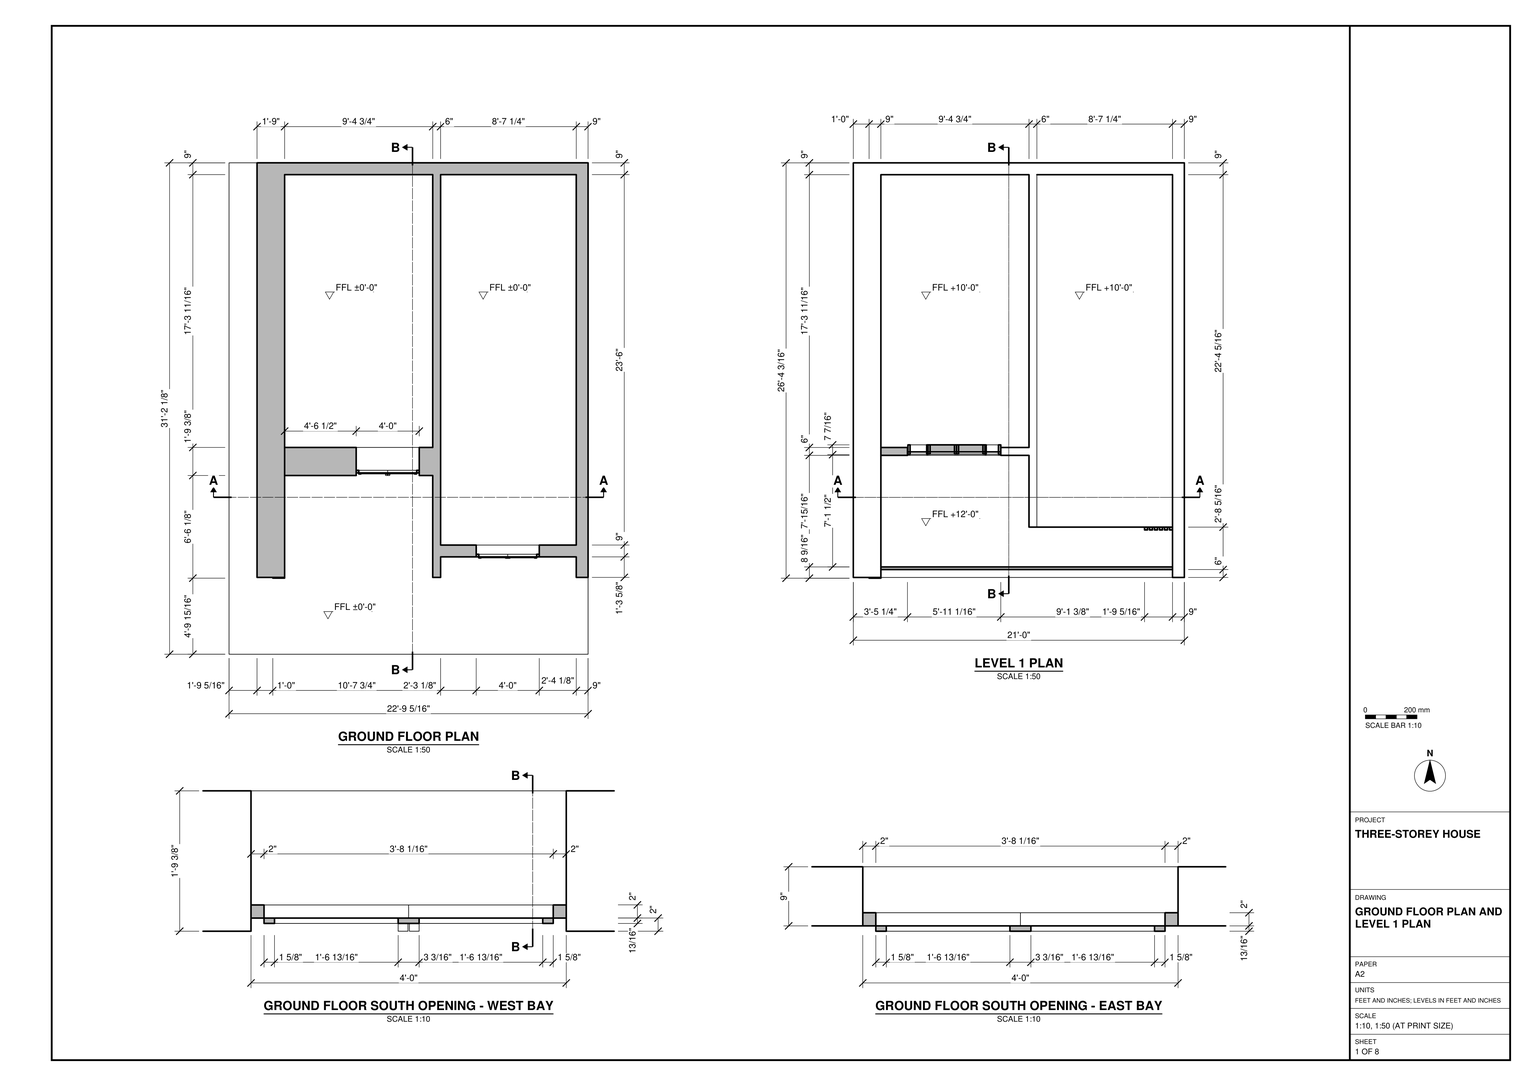
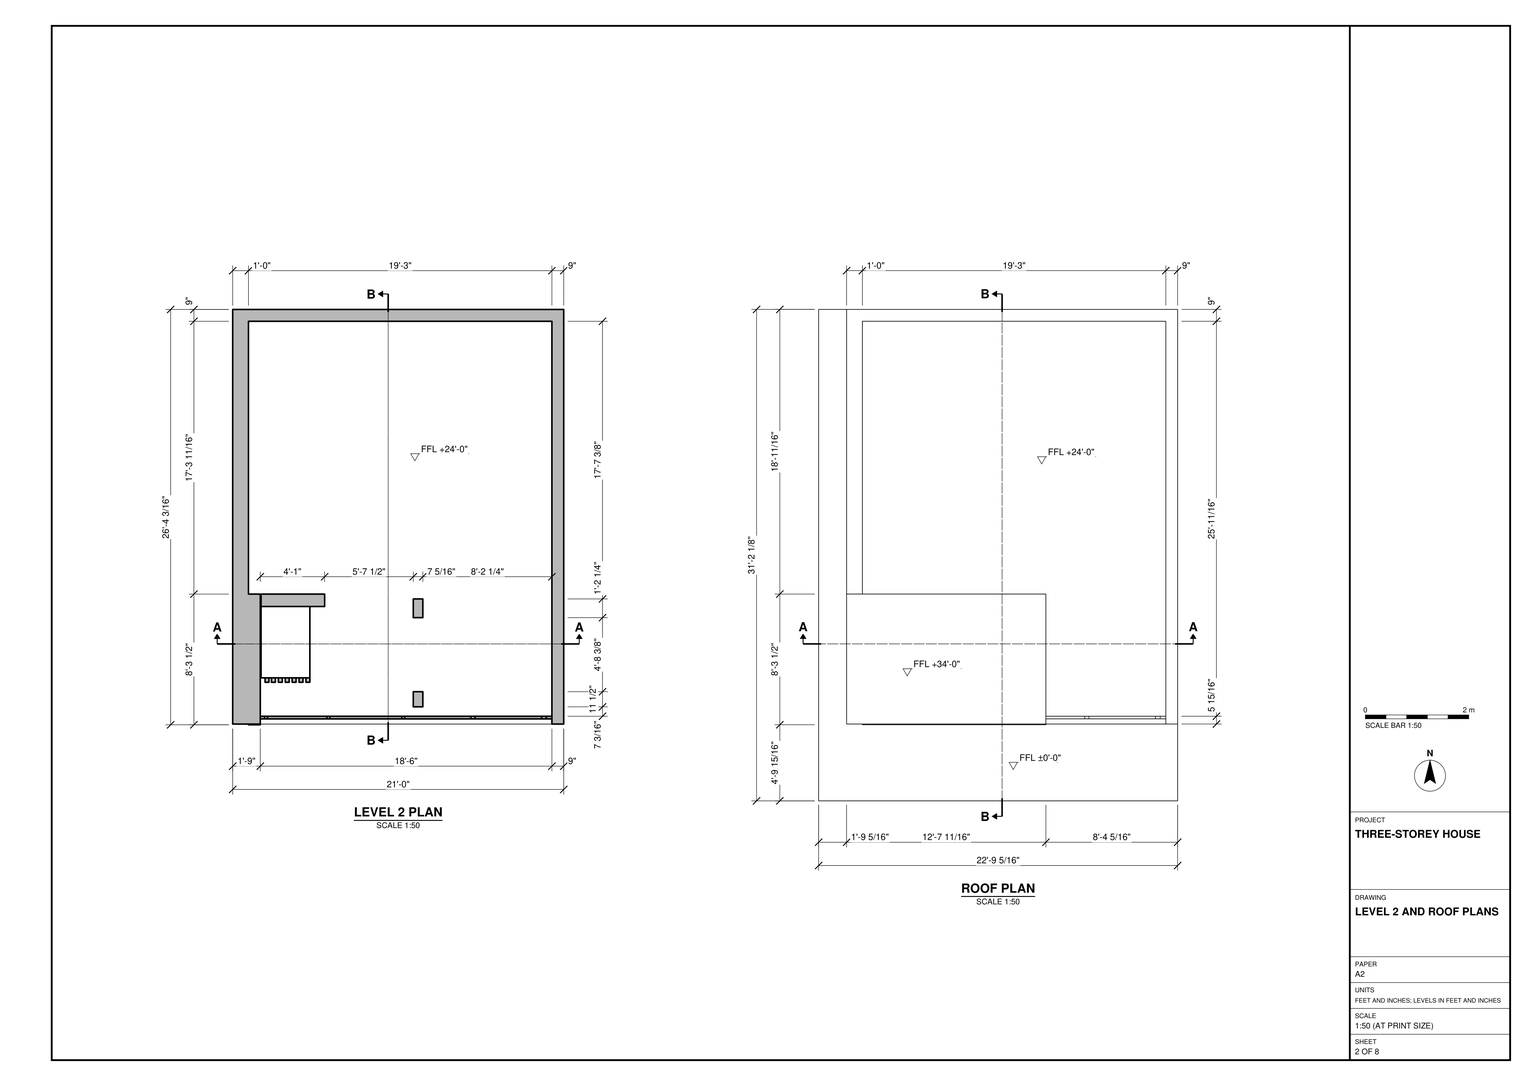
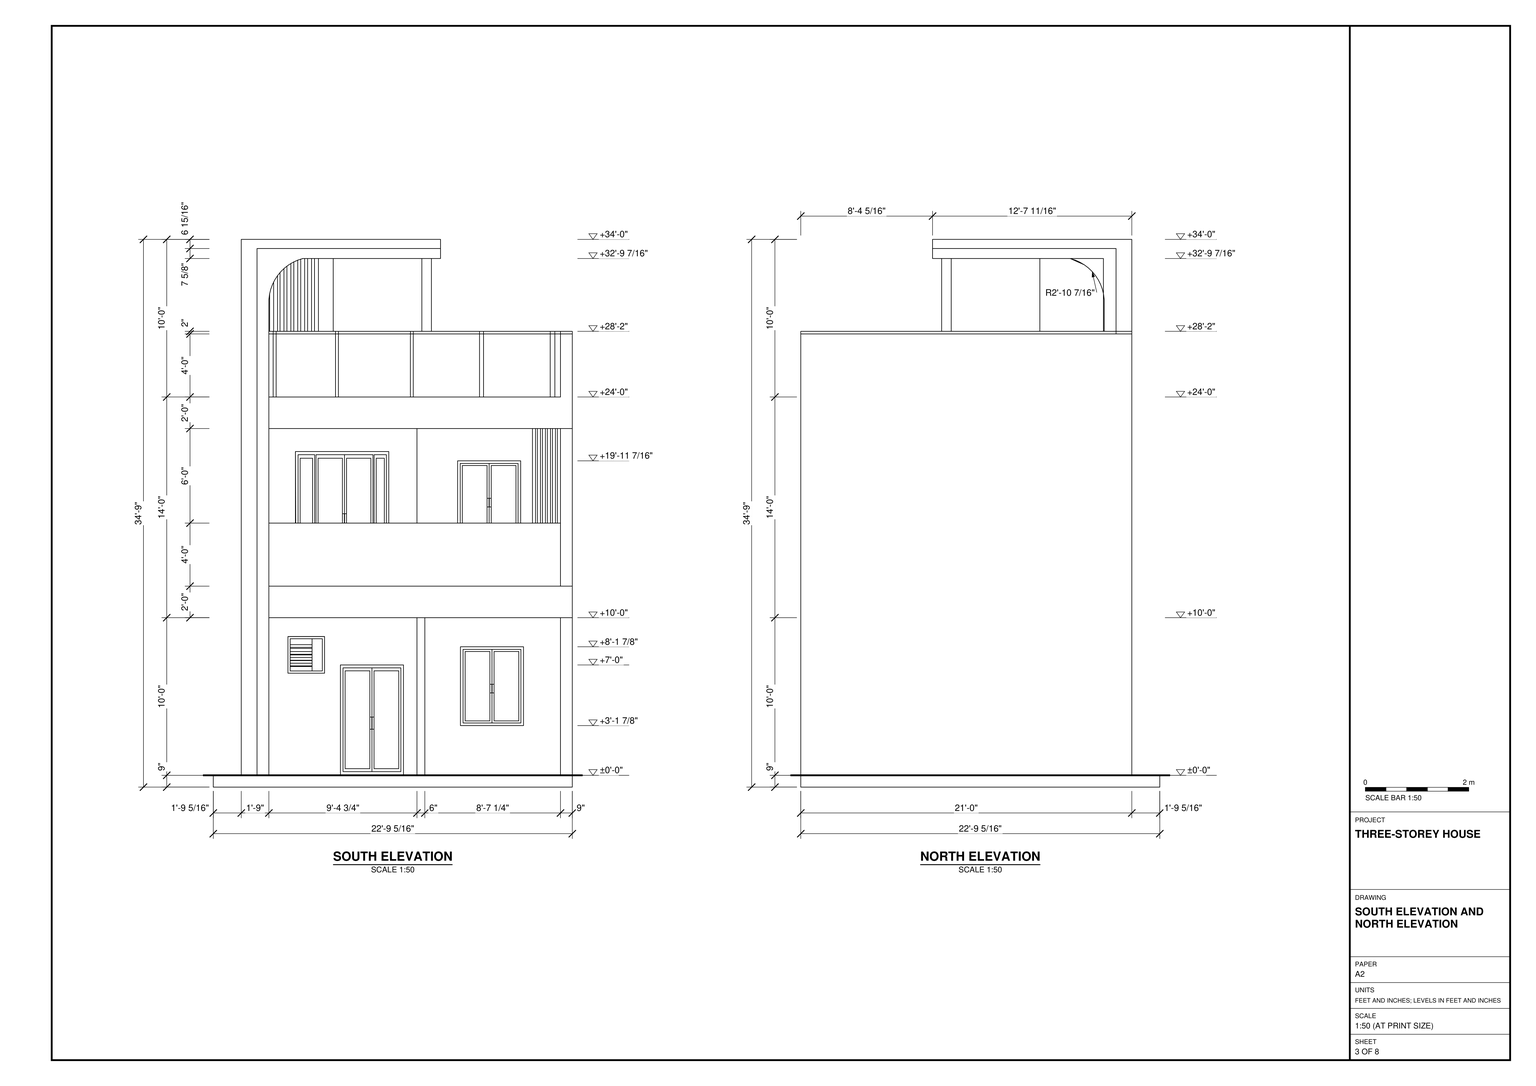
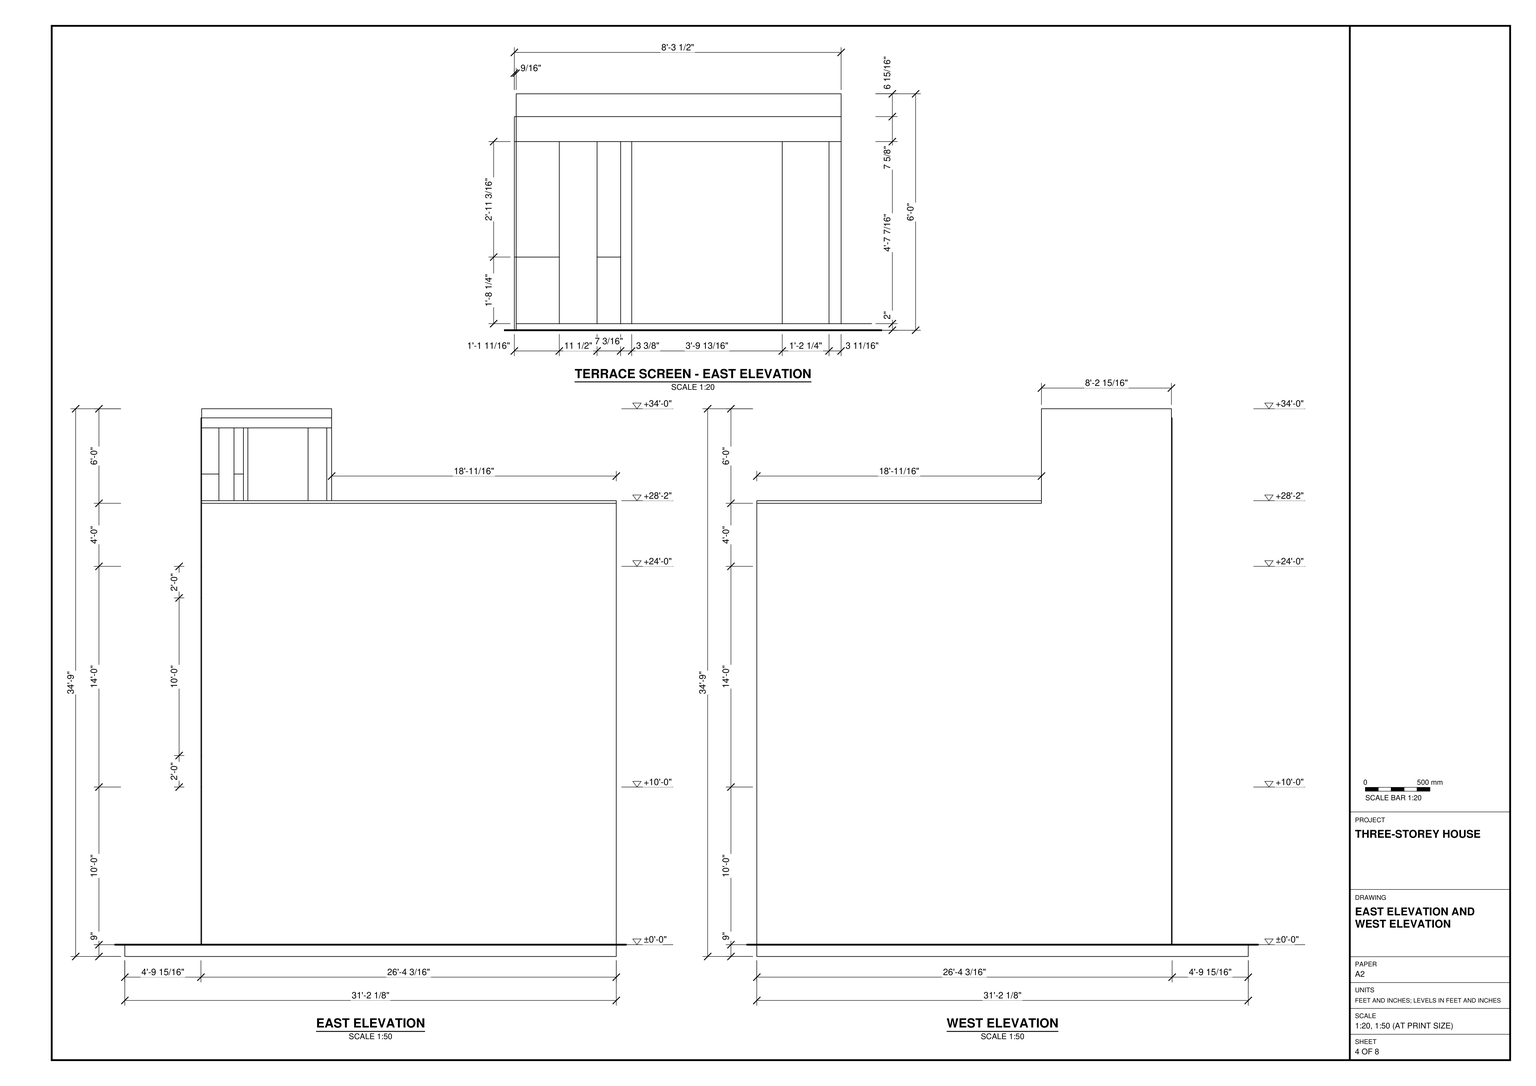
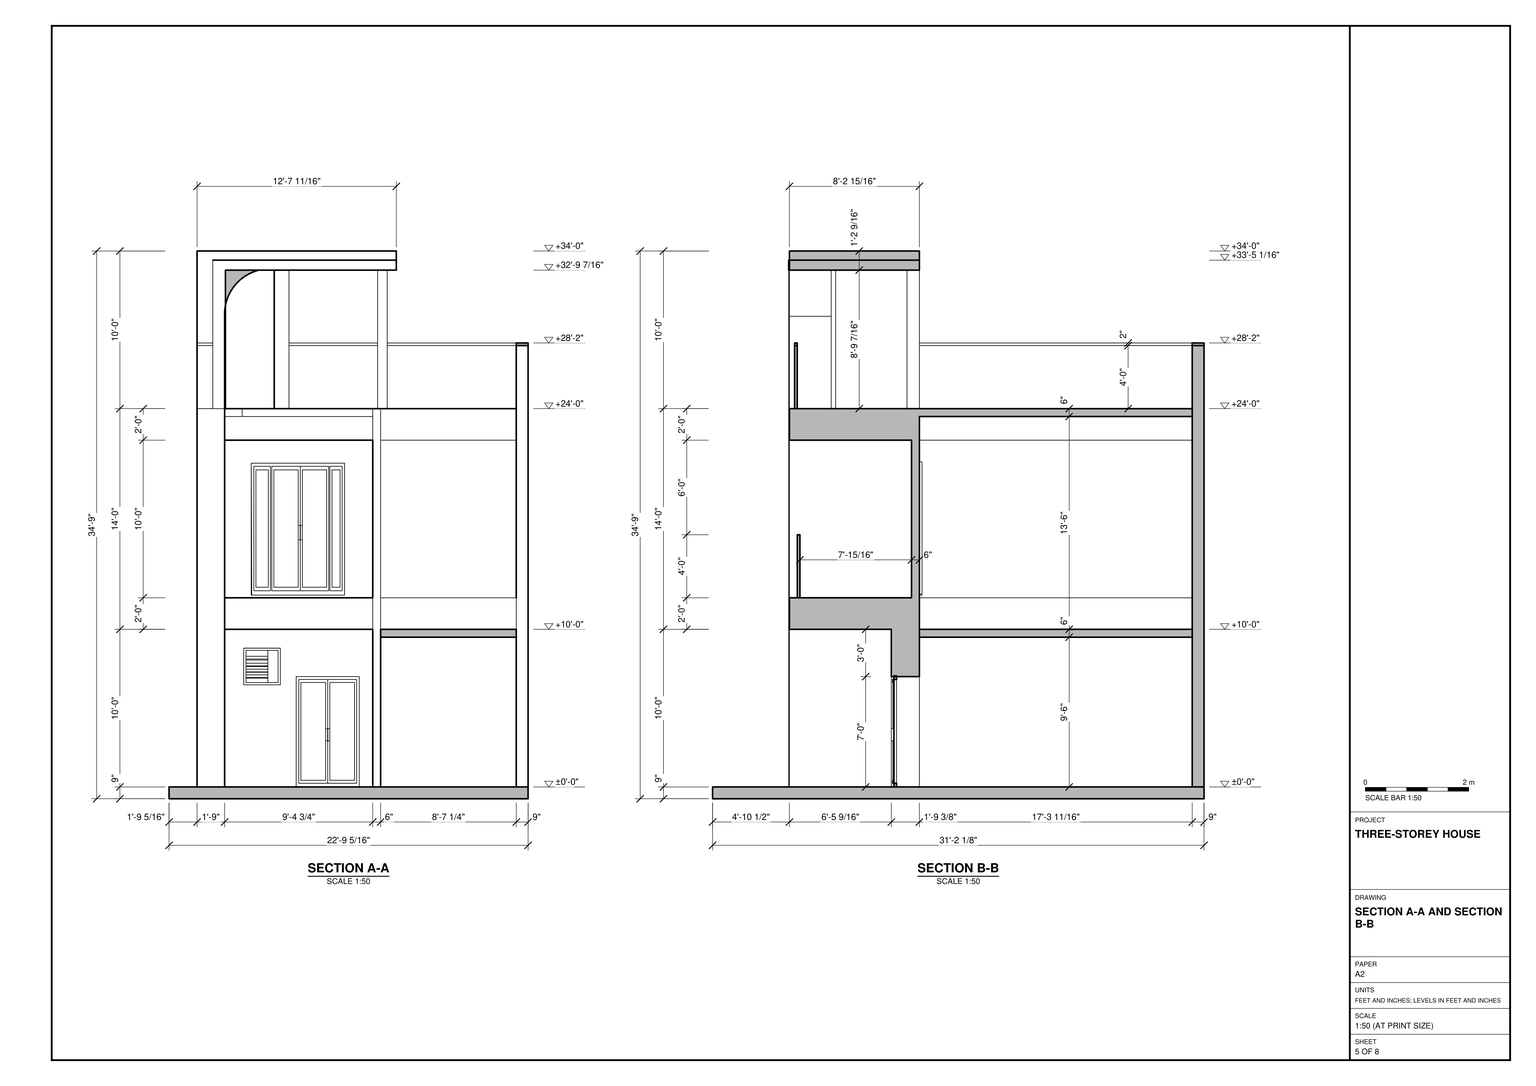
Build the house in SketchUp from task_files/diagram_01.pdf. Work in feet and inches. Including the base slab, the model measures 22'-9 5/16" east to west, 31'-2 1/8" north to south and 34'-9" high. Set the finished floor levels at ±0'-0", +10'-0" and +24'-0", with the front balcony floor at +12'-0".

Start with the projecting base slab. Lay out the two ground-floor bays with the west bay set farther back from the south slab edge than the east bay. Follow the wall thicknesses on each plan, including the 6" dividing wall and the thicker west wall. Fit the south openings with their frames and panel divisions. Include the small louvred opening beside the ground-floor door, the solid balcony front and the vertical screen at the east end of the balcony.

Follow the roof plan for the open terrace and the partial flat canopy over its southwest corner. Model the terrace guard, canopy supports and curved transition beneath the canopy as shown in elevation. Keep walls, slabs, roof elements and each furniture or joinery piece shown in separate groups or components, and use components for repeated parts. Any decor or loose items shown may be represented by suitable library components. Save one SketchUp model as output_files/three_storey_house_with_a_balcony_and_roof_terrace.skp.

# SketchUp Ruby script. Lengths in inches.
U = 1.inch
M = Sketchup.active_model
def pt(a) = Geom::Point3d.new(a.map { |v| v * U })
def face(e, loops, mat)
  f = e.add_face(loops[0].map { |a| pt(a) })
  loops[1..].each { |l| e.add_face(l.map { |a| pt(a) }).erase! }
  f.material = f.back_material = mat if mat
  f
end
# faces: each face lists its corners as indices into pts; further lists are holes
def faces(e, pts, list, mat = nil) = list.each { |f| face(e, (f[0].is_a?(Array) ? f : [f]).map { |l| l.map { |i| pts[i] } }, mat) }
# xy, xz, yz: faces in a plane at the given z, y or x. An outline is a flat list of corners, or four numbers for a rectangle; further outlines are holes
def ring(l) = l.size == 4 ? [[l[0], l[1]], [l[2], l[1]], [l[2], l[3]], [l[0], l[3]]] : l.each_slice(2).to_a
def flat(e, list, mat, &to3) = list.each { |f| face(e, (f[0].is_a?(Array) ? f : [f]).map { |l| ring(l).map { |u, v| to3.(u, v) } }, mat) }
def xy(e, z, list, mat = nil) = flat(e, list, mat) { |x, y| [x, y, z] }
def xz(e, y, list, mat = nil) = flat(e, list, mat) { |x, z| [x, y, z] }
def yz(e, x, list, mat = nil) = flat(e, list, mat) { |y, z| [x, y, z] }
def lines(e, pts, list) = list.each { |a, b| e.add_line(pt(pts[a]), pt(pts[b])) }
# prism: a flat outline (further loops are holes) pulled along v
def prism(e, loops, v, mat = nil)
  f = face(e, loops, mat); d = Geom::Vector3d.new(v.map { |x| x * U })
  f.pushpull(f.normal.samedirection?(d) ? d.length : -d.length)
end
def box(e, o, s, mat = nil) = prism(e, [[o, [o[0] + s[0], o[1], o[2]], [o[0] + s[0], o[1] + s[1], o[2]], [o[0], o[1] + s[1], o[2]]]], [0, 0, s[2]], mat)
def at(x, y, z, deg = 0) = Geom::Transformation.translation(pt([x, y, z])) * Geom::Transformation.rotation(ORIGIN, Z_AXIS, deg.degrees)
def axes(o, x, y, z) = Geom::Transformation.new([*x, 0, *y, 0, *z, 0, *pt(o).to_a, 1])
def part(name) = M.definitions.add(name)
# library, detail: a bought-in or finely detailed component or shape, given as its bounding box
def library(name, o, s) = part(name).tap { |d| box(d.entities, o, s) }
def detail(e, o, s) = box(e.add_group.entities, o, s)
def put(e, d, t, mat = nil) = e.add_instance(d, t).tap { |i| i.material = mat if mat }
def group(e, t, mat = nil) = e.add_group.tap { |g| g.transformation = t; g.material = mat if mat }.entities
root = M.entities
M.materials.add("[Blacktop Old 01]").color = [132, 136, 139]
M.materials.add("[Color A08]").color = [102, 0, 0]
M.materials.add("[Color L03]").color = [216, 169, 178]
M.materials.add("[Color L03]1").color = [227, 174, 178]
M.materials.add("[Color L11]").color = [153, 0, 76]
M.materials.add("[Color M00]").color = [255, 255, 255]
M.materials.add("[Color M05]").color = [114, 114, 114]
M.materials.add("[Color M07]").color = [58, 58, 58]
M.materials.add("[Metal Corrugated Shiny]").color = [215, 193, 104]
M.materials.add("[Metal Seamed]").color = [118, 119, 115]
M.materials.add("[Stone Brushed Khaki]").color = [226, 128, 133]
M.materials.add("[Translucent Glass Blue]").color = [100, 149, 237]
M.materials["[Translucent Glass Blue]"].alpha = 0.5
M.materials.add("[Translucent Glass Dark Green]").color = [62, 91, 5]
M.materials["[Translucent Glass Dark Green]"].alpha = 0.5
M.materials.add("[Translucent Glass Gray]").color = [128, 128, 128]
M.materials["[Translucent Glass Gray]"].alpha = 0.5
M.materials.add("[Wood Bamboo]").color = [141, 105, 43]
c1 = part("Group\#1")
xy(c1.entities,0,[[0,2,48,4]],"[Wood Bamboo]")
xy(c1.entities,1.98,[[1.98,1.1875,24,2],[24,1.1875,46.02,2],[1.98,2,24,4],[24,2,46.02,4]],"[Wood Bamboo]")
xy(c1.entities,3.58,[[3.58,1.1875,22.4,2],[25.6,1.1875,44.42,2]],"[Wood Bamboo]")
xy(c1.entities,24.88,[[22.4,1.1875,23.9,2],[23.9,1.1875,24,2],[24,1.1875,24.12,2],[24.12,1.1875,25.6,2]])
xy(c1.entities,24.88,[[22.4,0,23.9,1.1875],[24.12,0,25.6,1.1875]],"[Metal Corrugated Shiny]")
xy(c1.entities,31.44,[[22.4,1.1875,23.9,2],[23.9,1.1875,24,2],[24,1.1875,24.12,2],[24.12,1.1875,25.6,2]])
xy(c1.entities,31.44,[[22.4,0,23.9,1.1875],[24.12,0,25.6,1.1875]],"[Metal Corrugated Shiny]")
xy(c1.entities,56.42,[[3.58,1.1875,22.4,2],[25.6,1.1875,44.42,2]],"[Wood Bamboo]")
xy(c1.entities,58.02,[[1.98,1.1875,24,2],[24,1.1875,46.02,2],[1.98,2,24,4],[24,2,46.02,4]],"[Wood Bamboo]")
xy(c1.entities,60,[[0,2,48,4]],"[Wood Bamboo]")
xz(c1.entities,0,[[22.4,24.88,23.9,31.44],[24.12,24.88,25.6,31.44]],"[Metal Corrugated Shiny]")
xz(c1.entities,1.1875,[[1.98,1.98,24,1.98,24,24.88,22.4,24.88,22.4,3.58,3.58,3.58,3.58,56.42,22.4,56.42,22.4,31.44,24,31.44,24,58.02,1.98,58.02],[24,1.98,46.02,1.98,46.02,58.02,24,58.02,24,31.44,25.6,31.44,25.6,56.42,44.42,56.42,44.42,3.58,25.6,3.58,25.6,24.88,24,24.88]],"[Wood Bamboo]")
xz(c1.entities,2,[[22.4,24.88,23.9,31.44],[23.9,24.88,24,31.44],[24,24.88,24.12,31.44],[24.12,24.88,25.6,31.44]])
xz(c1.entities,2,[[3.58,3.58,22.4,56.42],[25.6,3.58,44.42,56.42]],"[Translucent Glass Dark Green]")
xz(c1.entities,2,[[[0,0,48,60],[1.98,1.98,46.02,58.02]],[[1.98,1.98,46.02,58.02],[3.58,3.58,3.58,56.42,22.4,56.42,22.4,31.44,25.6,31.44,25.6,56.42,44.42,56.42,44.42,3.58,25.6,3.58,25.6,24.88,22.4,24.88,22.4,3.58]]],"[Wood Bamboo]")
xz(c1.entities,4,[[[0,0,48,60],[1.98,1.98,46.02,58.02]]],"[Wood Bamboo]")
yz(c1.entities,0,[[2,0,4,60]],"[Wood Bamboo]")
yz(c1.entities,1.98,[[1.1875,1.98,2,58.02],[2,1.98,4,58.02]],"[Wood Bamboo]")
yz(c1.entities,3.58,[[1.1875,3.58,2,56.42]],"[Wood Bamboo]")
yz(c1.entities,22.4,[[0,24.88,2,31.44]],"[Metal Corrugated Shiny]")
yz(c1.entities,22.4,[[1.1875,3.58,2,24.88],[1.1875,31.44,2,56.42]],"[Wood Bamboo]")
yz(c1.entities,23.9,[[0,24.88,2,31.44]],"[Metal Corrugated Shiny]")
yz(c1.entities,24.12,[[0,24.88,2,31.44]],"[Metal Corrugated Shiny]")
yz(c1.entities,25.6,[[0,24.88,2,31.44]],"[Metal Corrugated Shiny]")
yz(c1.entities,25.6,[[1.1875,3.58,2,24.88],[1.1875,31.44,2,56.42]],"[Wood Bamboo]")
yz(c1.entities,44.42,[[1.1875,3.58,2,56.42]],"[Wood Bamboo]")
yz(c1.entities,46.02,[[1.1875,1.98,2,58.02],[2,1.98,4,58.02]],"[Wood Bamboo]")
yz(c1.entities,48,[[2,0,4,60]],"[Wood Bamboo]")
xy(root,0,[[0,0,273.3125,374.125]],"[Stone Brushed Khaki]")
xy(root,9,[[33.3125,57.9375,42.3125,58.5],[21.3125,58.5,33.3125,374.125],[33.3125,58.5,33.3125,374.125,273.3125,374.125,273.3125,58.5,264.3125,58.5,264.3125,365.125,161.0625,365.125,161.0625,58.5,155.0625,58.5,155.0625,136.0625,144.79,136.0625,144.79,157.4375,155.0625,157.4375,155.0625,365.125,42.3125,365.125,42.3125,58.5],[161.0625,74.125,264.3125,83.125],[161.0625,83.125,264.3125,365.125],
  [42.3125,136.0625,96.79,157.4375],[42.3125,157.4375,155.0625,365.125]])
xy(root,9,[[0,0,273.3125,0,273.3125,58.5,264.3125,58.5,264.3125,74.125,161.0625,74.125,161.0625,58.5,155.0625,58.5,155.0625,136.0625,144.79,136.0625,144.79,157.4375,96.79,157.4375,96.79,136.0625,42.3125,136.0625,42.3125,57.9375,33.3125,57.9375,33.3125,58.5,21.3125,58.5,21.3125,374.125,0,374.125]],"[Stone Brushed Khaki]")
xy(root,46.85,[[188.16,74.125,236.16,83.125]],"[Color M00]")
xy(root,86.74,[[56.84,136.0625,84.72,157.4375]])
xy(root,93,[[96.79,136.0625,144.79,157.4375]])
xy(root,106.85,[[188.16,74.125,236.16,83.125]],"[Color M00]")
xy(root,114.61,[[56.84,136.0625,84.72,157.4375]])
xy(root,123,[[161.0625,83.125,264.3125,365.125],[42.3125,157.4375,155.0625,365.125]])
xy(root,129,[[161.0625,83.125,264.3125,365.125],[42.3125,157.4375,155.0625,365.125]])
xy(root,129,[[42.3125,58.5,155.0625,136.0625],[161.0625,58.5,264.3125,74.125]],"[Color L03]")
xy(root,153,[[42.3125,58.5,264.3125,64.5],[42.3125,64.5,264.3125,66.5],[42.3125,66.5,264.3125,66.5,264.3125,94.6875,262.01,94.6875,262.01,96.8125,260.5,96.8125,260.5,94.6875,258.19,94.6875,258.19,96.8125,256.6875,96.8125,256.6875,94.6875,254.38,94.6875,254.38,96.8125,252.875,96.8125,252.875,94.6875,250.57,94.6875,250.57,96.8125,249.0625,96.8125,249.0625,94.6875,246.76,94.6875,246.76,96.8125,245.3125,96.8125,245.3125,94.6875,243.01,94.6875,243.01,96.8125,155.0625,96.8125,155.0625,151.4375,42.3125,151.4375]])
xy(root,153,[[243.01,94.6875,245.3125,96.8125],[246.76,94.6875,249.0625,96.8125],[250.57,94.6875,252.875,96.8125],[254.38,94.6875,256.6875,96.8125],[258.19,94.6875,260.5,96.8125],
  [262.01,94.6875,264.3125,96.8125]],"[Color M00]")
xy(root,154.99,[[62.54,151.4375,133.6,157.4375]])
xy(root,188.42,[[186.01,96.8125,234.01,117.4375]],"[Color M00]")
xy(root,201,[[42.3125,64.5,264.3125,66.5]],"[Metal Seamed]")
xy(root,248.42,[[186.01,96.8125,234.01,117.4375]],"[Color M00]")
xy(root,255.49,[[62.54,151.4375,133.6,157.4375]])
xy(root,273,[[42.3125,58.5,42.3125,151.4375,155.0625,151.4375,155.0625,96.8125,243.01,96.8125,243.01,94.6875,245.3125,94.6875,245.3125,96.8125,246.76,96.8125,246.76,94.6875,249.0625,94.6875,249.0625,96.8125,250.57,96.8125,250.57,94.6875,252.875,94.6875,252.875,96.8125,254.38,96.8125,254.38,94.6875,256.6875,94.6875,256.6875,96.8125,258.19,96.8125,258.19,94.6875,260.5,94.6875,260.5,96.8125,262.01,96.8125,262.01,94.6875,264.3125,94.6875,264.3125,58.5]],"[Color L03]")
xy(root,273,[[243.01,94.6875,245.3125,96.8125],[246.76,94.6875,249.0625,96.8125],[250.57,94.6875,252.875,96.8125],[254.38,94.6875,256.6875,96.8125],[258.19,94.6875,260.5,96.8125],
  [262.01,94.6875,264.3125,96.8125]],"[Color M00]")
xy(root,291,[[42.3125,157.4375,155.0625,365.125]])
xy(root,297,[[42.3125,62.4375,45.58,64.4375],[45.58,62.4375,47.87,64.4375],[47.87,62.4375,93.0625,64.4375],[93.0625,62.4375,95.25,64.4375],[95.25,62.4375,150.0625,64.4375],
  [152.25,62.4375,202.6875,64.4375],[202.6875,62.4375,205.75,64.4375],[205.75,62.4375,256.5,64.4375],[256.5,62.4375,260.03,64.4375],[260.03,62.4375,264.3125,64.4375],
  [45.95,90.3,48.93,93.68],[50.82,90.3,53.81,93.68],[56.07,90.3,59.06,93.68],[61.32,90.3,64.31,93.68],[66.57,90.3,69.56,93.68],
  [71.82,90.3,74.81,93.68],[77.07,90.3,80.06,93.68],[42.92,93.68,80.06,147.99],[158.78,139.51,161.0625,153.75],[161.0625,139.51,166.07,153.75],
  [42.92,147.99,91.31,157.4375]])
xy(root,297,[[[42.3125,64.4375,264.3125,64.4375,264.3125,365.125,33.3125,365.125,33.3125,157.4375,42.3125,157.4375],[45.95,90.3,45.95,93.68,42.92,93.68,42.92,157.4375,91.31,157.4375,91.31,147.99,80.06,147.99,80.06,90.3,77.07,90.3,77.07,93.68,74.81,93.68,74.81,90.3,71.82,90.3,71.82,93.68,69.56,93.68,69.56,90.3,66.57,90.3,66.57,93.68,64.31,93.68,64.31,90.3,61.32,90.3,61.32,93.68,59.06,93.68,59.06,90.3,56.07,90.3,56.07,93.68,53.81,93.68,53.81,90.3,50.82,90.3,50.82,93.68,48.93,93.68,48.93,90.3],[158.78,139.51,166.07,153.75],[158.78,71.625,166.07,83.125]]],"[Blacktop Old 01]")
xy(root,297,[[42.3125,58.5,264.3125,62.4375]],"[Metal Seamed]")
xy(root,345,[[42.3125,62.4375,45.58,64.4375]])
xy(root,345,[[264.3125,58.5,264.3125,365.125,33.3125,365.125,33.3125,157.4375,21.3125,157.4375,21.3125,374.125,273.3125,374.125,273.3125,58.5]],"[Color M07]")
xy(root,345,[[45.58,62.4375,47.87,64.4375],[47.87,62.4375,93.0625,64.4375],[93.0625,62.4375,95.25,64.4375],[95.25,62.4375,150.0625,64.4375],[150.0625,62.4375,152.25,64.4375],
  [152.25,62.4375,202.6875,64.4375],[202.6875,62.4375,205.75,64.4375],[205.75,62.4375,256.5,64.4375],[256.5,62.4375,260.03,64.4375],[260.03,62.4375,264.3125,64.4375]],"[Metal Seamed]")
xy(root,347,[[264.3125,58.5,273.3125,58.5,273.3125,374.125,21.3125,374.125,21.3125,157.4375,33.3125,157.4375,33.3125,365.125,264.3125,365.125]],"[Color M07]")
xy(root,347,[[42.3125,62.4375,45.58,64.4375],[45.58,62.4375,47.87,64.4375],[47.87,62.4375,93.0625,64.4375],[93.0625,62.4375,95.25,64.4375],[95.25,62.4375,150.0625,64.4375],
  [150.0625,62.4375,152.25,64.4375],[152.25,62.4375,202.6875,64.4375],[202.6875,62.4375,205.75,64.4375],[205.75,62.4375,256.5,64.4375],[256.5,62.4375,260.03,64.4375],
  [260.03,62.4375,264.3125,64.4375]],"[Metal Seamed]")
xy(root,402.45,[[68.23,57.9375,158.78,58.5],[158.78,57.9375,166.07,58.5],[166.07,57.9375,173,58.5],[68.23,58.5,68.23,90.3,69.56,90.3,69.56,93.68,71.82,93.68,71.82,90.3,74.81,90.3,74.81,93.68,77.07,93.68,77.07,90.3,80.06,90.3,80.06,147.99,91.31,147.99,91.31,157.4375,158.78,157.4375,158.78,139.51,166.07,139.51,166.07,157.4375,173,157.4375,173,58.5,166.07,58.5,166.07,83.125,158.78,83.125,158.78,58.5],[158.78,58.5,166.07,71.625],
  [158.78,71.625,166.07,83.125],[45.95,90.3,48.93,93.68],[50.82,90.3,53.81,93.68],[56.07,90.3,59.06,93.68],[61.32,90.3,64.31,93.68],
  [66.57,90.3,68.23,93.68],[68.23,90.3,69.56,93.68],[71.82,90.3,74.81,93.68],[77.07,90.3,80.06,93.68],[42.92,93.68,68.23,147.99],
  [68.23,93.68,80.06,147.99],[158.78,139.51,166.07,153.75],[42.92,147.99,68.23,157.4375],[68.23,147.99,91.31,157.4375],[158.78,153.75,166.07,157.4375]])
xy(root,410.06,[[33.3125,57.9375,173,58.5],[33.3125,58.5,173,157.4375]])
xy(root,417,[[21.3125,58.5,173,157.4375]],"[Color L03]1")
xz(root,0,[[0,0,273.3125,9]],"[Stone Brushed Khaki]")
xz(root,57.9375,[[33.3125,9,42.3125,9,42.3125,367.28,42.33,371.22,42.81,375.13,43.72,378.97,45.07,382.67,46.83,386.2,48.98,389.5,51.5,392.53,54.35,395.26,57.49,397.64,60.875,399.65,64.47,401.26,68.23,402.45,173,402.45,173,410.06,33.3125,410.06]],"[Color L03]")
xz(root,58.5,[[33.3125,9,33.3125,410.06,173,410.06,173,402.45,68.23,402.45,64.47,401.26,60.875,399.65,57.49,397.64,54.35,395.26,51.5,392.53,48.98,389.5,46.83,386.2,45.07,382.67,43.72,378.97,42.81,375.13,42.33,371.22,42.3125,367.28,42.3125,9]])
xz(root,58.5,[[21.3125,9,33.3125,9,33.3125,410.06,173,410.06,173,417,21.3125,417],[264.3125,153,273.3125,273]],"[Color L03]")
xz(root,58.5,[[155.0625,9,161.0625,129],[264.3125,9,273.3125,129]],"[Color L03]1")
xz(root,58.5,[[42.3125,129,273.3125,153],[42.3125,273,273.3125,273,273.3125,345,264.3125,345,264.3125,297,42.3125,297]],"[Color L11]")
xz(root,58.5,[[264.3125,345,273.3125,347]],"[Color M07]")
xz(root,62.4375,[[45.58,297,47.87,345],[93.0625,297,95.25,345],[150.0625,297,152.25,345],[202.6875,297,205.75,345],[256.5,297,260.03,345],
  [42.3125,345,45.58,347],[45.58,345,47.87,347],[47.87,345,93.0625,347],[93.0625,345,95.25,347],[95.25,345,150.0625,347],
  [150.0625,345,152.25,347],[152.25,345,202.6875,347],[202.6875,345,205.75,347],[205.75,345,256.5,347],[256.5,345,260.03,347],
  [260.03,345,264.3125,347]],"[Metal Seamed]")
xz(root,62.4375,[[42.3125,297,45.58,345],[47.87,297,93.0625,345],[95.25,297,150.0625,345],[152.25,297,202.6875,345],[205.75,297,256.5,345],
  [260.03,297,264.3125,345]],"[Translucent Glass Gray]")
xz(root,64.4375,[[45.58,297,47.87,345],[93.0625,297,95.25,345],[150.0625,297,152.25,345],[202.6875,297,205.75,345],[256.5,297,260.03,345],
  [42.3125,345,45.58,347],[45.58,345,47.87,347],[47.87,345,93.0625,347],[93.0625,345,95.25,347],[95.25,345,150.0625,347],
  [150.0625,345,152.25,347],[152.25,345,202.6875,347],[202.6875,345,205.75,347],[205.75,345,256.5,347],[256.5,345,260.03,347],
  [260.03,345,264.3125,347]],"[Metal Seamed]")
xz(root,64.4375,[[42.3125,297,45.58,345],[47.87,297,93.0625,345],[95.25,297,150.0625,345],[152.25,297,202.6875,345],[205.75,297,256.5,345],
  [260.03,297,264.3125,345]],"[Translucent Glass Gray]")
xz(root,64.5,[[42.3125,153,264.3125,201]],"[Translucent Glass Gray]")
xz(root,66.5,[[42.3125,153,264.3125,201]],"[Translucent Glass Gray]")
xz(root,71.625,[[158.78,297,166.07,402.45]],"[Color L03]1")
xz(root,74.125,[[[161.0625,9,264.3125,129],[188.16,46.85,236.16,106.85]]],"[Color L03]")
xz(root,83.125,[[[161.0625,9,264.3125,123],[188.16,46.85,236.16,106.85]],[161.0625,123,264.3125,129]])
xz(root,83.125,[[158.78,297,166.07,402.45]],"[Color L03]1")
xz(root,90.3,[[45.95,297,48.93,402.45],[50.82,297,53.81,402.45],[56.07,297,59.06,402.45],[61.32,297,64.31,402.45],[66.57,297,69.56,402.45],
  [71.82,297,74.81,402.45],[77.07,297,80.06,402.45]],"[Color M05]")
xz(root,93.68,[[45.95,297,48.93,402.45],[50.82,297,53.81,402.45],[56.07,297,59.06,402.45],[61.32,297,64.31,402.45],[66.57,297,69.56,402.45],
  [71.82,297,74.81,402.45],[77.07,297,80.06,402.45]])
xz(root,93.68,[[42.92,297,45.95,402.45],[48.93,297,50.82,402.45],[53.81,297,56.07,402.45],[59.06,297,61.32,402.45],[64.31,297,66.57,402.45],
  [69.56,297,71.82,402.45],[74.81,297,77.07,402.45]],"[Color M05]")
xz(root,94.6875,[[243.01,153,245.3125,273],[246.76,153,249.0625,273],[250.57,153,252.875,273],[254.38,153,256.6875,273],[258.19,153,260.5,273],
  [262.01,153,264.3125,273]],"[Color M05]")
xz(root,96.8125,[[[155.0625,153,243.01,273],[186.01,188.42,234.01,248.42]]],"[Color L03]")
xz(root,96.8125,[[243.01,153,245.3125,273],[246.76,153,249.0625,273],[250.57,153,252.875,273],[254.38,153,256.6875,273],[258.19,153,260.5,273],
  [262.01,153,264.3125,273]],"[Color M00]")
xz(root,96.8125,[[245.3125,153,246.76,273],[249.0625,153,250.57,273],[252.875,153,254.38,273],[256.6875,153,258.19,273],[260.5,153,262.01,273]],"[Color M05]")
xz(root,117.4375,[[186.01,188.42,234.01,248.42]],"[Color M00]")
xz(root,136.0625,[[[42.3125,9,96.79,9,96.79,93,144.79,93,144.79,9,155.0625,9,155.0625,129,42.3125,129],[56.84,86.74,84.72,114.61]]],"[Color L03]")
xz(root,139.51,[[158.78,297,166.07,402.45]],"[Color L03]1")
xz(root,147.99,[[42.92,297,80.06,402.45]])
xz(root,147.99,[[80.06,297,91.31,402.45]],"[Color L03]1")
xz(root,151.4375,[[[42.3125,153,155.0625,273],[62.54,154.99,133.6,255.49]]],"[Color L03]")
xz(root,153.75,[[158.78,297,166.07,402.45]],"[Color L03]1")
xz(root,157.4375,[[[42.3125,9,42.3125,123,155.0625,123,155.0625,9,144.79,9,144.79,93,96.79,93,96.79,9],[56.84,86.74,84.72,114.61]],[42.3125,123,155.0625,129],[42.3125,129,155.0625,153],[[42.3125,153,155.0625,273],[62.54,154.99,133.6,255.49]],[42.3125,273,155.0625,291]])
xz(root,157.4375,[[33.3125,297,33.3125,410.06,173,410.06,173,402.45,42.92,402.45,42.92,375.62,42.81,375.13,42.33,371.22,42.3125,367.28,42.3125,297],[42.92,297,42.92,375.62,43.72,378.97,45.07,382.67,46.83,386.2,48.98,389.5,51.5,392.53,54.35,395.26,57.49,397.64,60.875,399.65,64.47,401.26,68.23,402.45,91.31,402.45,91.31,297],[21.3125,347,21.3125,417,173,417,173,410.06,33.3125,410.06,33.3125,347],[42.92,375.62,42.92,402.45,68.23,402.45,64.47,401.26,60.875,399.65,57.49,397.64,54.35,395.26,51.5,392.53,48.98,389.5,46.83,386.2,45.07,382.67,43.72,378.97]],"[Color L03]1")
xz(root,157.4375,[[21.3125,345,33.3125,347]],"[Color M07]")
xz(root,365.125,[[42.3125,9,155.0625,123],[161.0625,9,264.3125,123],[42.3125,123,52.25,129],[52.25,123,155.0625,129],[161.0625,123,178.375,129],
  [178.375,123,264.3125,129],[42.3125,129,155.0625,153],[161.0625,129,264.3125,153],[42.3125,153,155.0625,273],[161.0625,153,264.3125,273],
  [42.3125,273,155.0625,291],[161.0625,273,264.3125,297],[42.3125,291,55.6875,297],[55.6875,291,155.0625,297]])
xz(root,365.125,[[33.3125,297,264.3125,345]],"[Color L03]1")
xz(root,365.125,[[33.3125,345,264.3125,347]],"[Color M07]")
xz(root,374.125,[[21.3125,9,273.3125,345]],"[Color L03]")
xz(root,374.125,[[21.3125,345,33.3125,347],[33.3125,345,273.3125,347]],"[Color M07]")
xz(root,374.125,[[0,0,273.3125,9]],"[Stone Brushed Khaki]")
yz(root,0,[[0,0,374.125,9]],"[Stone Brushed Khaki]")
yz(root,21.3125,[[58.5,9,58.5,417,157.4375,417,157.4375,345,374.125,345,374.125,9]],"[Color L03]")
yz(root,21.3125,[[157.4375,345,374.125,347]],"[Color M07]")
yz(root,33.3125,[[57.9375,9,58.5,410.06]])
yz(root,33.3125,[[157.4375,297,365.125,345]],"[Color L03]1")
yz(root,33.3125,[[157.4375,345,365.125,347]],"[Color M07]")
yz(root,42.3125,[[57.9375,9,58.5,129],[136.0625,9,157.4375,129],[157.4375,9,365.125,123],[157.4375,123,365.125,129],[57.9375,129,58.5,153],
  [58.5,129,157.4375,153],[157.4375,129,365.125,153],[57.9375,153,58.5,273],[64.5,153,66.5,201],[151.4375,153,157.4375,273],
  [157.4375,153,365.125,273],[57.9375,273,58.5,297],[58.5,273,151.4375,297],[151.4375,273,157.4375,297],[157.4375,273,365.125,291],
  [57.9375,297,58.5,367.28],[62.4375,297,64.4375,345],[62.4375,345,64.4375,347]])
yz(root,42.3125,[[58.5,153,64.5,153,64.5,201,66.5,201,66.5,153,151.4375,153,151.4375,273,58.5,273]],"[Color L03]")
yz(root,42.3125,[[58.5,9,136.0625,129],[58.5,297,62.4375,297,62.4375,347,64.4375,347,64.4375,297,157.4375,297,157.4375,367.28,58.5,367.28]],"[Color L03]1")
yz(root,42.92,[[93.68,297,147.99,402.45],[147.99,297,157.4375,402.45]])
yz(root,45.58,[[62.4375,345,64.4375,347]])
yz(root,45.58,[[62.4375,297,64.4375,345]],"[Metal Seamed]")
yz(root,45.95,[[90.3,297,93.68,402.45]],"[Color M05]")
yz(root,47.87,[[62.4375,297,64.4375,345],[62.4375,345,64.4375,347]],"[Metal Seamed]")
yz(root,48.93,[[90.3,297,93.68,402.45]],"[Color M05]")
yz(root,50.82,[[90.3,297,93.68,402.45]],"[Color M05]")
yz(root,53.81,[[90.3,297,93.68,402.45]],"[Color M05]")
yz(root,56.07,[[90.3,297,93.68,402.45]],"[Color M05]")
yz(root,56.84,[[136.0625,86.74,157.4375,114.61]])
yz(root,59.06,[[90.3,297,93.68,402.45]],"[Color M05]")
yz(root,61.32,[[90.3,297,93.68,402.45]],"[Color M05]")
yz(root,62.54,[[151.4375,154.99,157.4375,255.49]])
yz(root,64.31,[[90.3,297,93.68,402.45]],"[Color M05]")
yz(root,66.57,[[90.3,297,93.68,402.45]],"[Color M05]")
yz(root,69.56,[[90.3,297,93.68,402.45]],"[Color M05]")
yz(root,71.82,[[90.3,297,93.68,402.45]],"[Color M05]")
yz(root,74.81,[[90.3,297,93.68,402.45]],"[Color M05]")
yz(root,77.07,[[90.3,297,93.68,402.45]],"[Color M05]")
yz(root,80.06,[[93.68,297,147.99,402.45]],"[Color L03]1")
yz(root,80.06,[[90.3,297,93.68,402.45]],"[Color M05]")
yz(root,84.72,[[136.0625,86.74,157.4375,114.61]])
yz(root,91.31,[[147.99,297,157.4375,402.45]],"[Color L03]1")
yz(root,93.0625,[[62.4375,297,64.4375,345],[62.4375,345,64.4375,347]],"[Metal Seamed]")
yz(root,95.25,[[62.4375,297,64.4375,345],[62.4375,345,64.4375,347]],"[Metal Seamed]")
yz(root,96.79,[[136.0625,9,157.4375,93]])
yz(root,133.6,[[151.4375,154.99,157.4375,255.49]])
yz(root,144.79,[[136.0625,9,157.4375,93]])
yz(root,150.0625,[[62.4375,297,64.4375,345],[62.4375,345,64.4375,347]],"[Metal Seamed]")
yz(root,152.25,[[62.4375,297,64.4375,345],[62.4375,345,64.4375,347]],"[Metal Seamed]")
yz(root,155.0625,[[157.4375,9,365.125,123],[157.4375,123,365.125,129],[157.4375,129,365.125,153],[157.4375,153,365.125,273],[157.4375,273,365.125,291]])
yz(root,155.0625,[[58.5,9,136.0625,129],[96.8125,153,151.4375,273]],"[Color L03]")
yz(root,158.78,[[71.625,297,83.125,402.45],[139.51,297,153.75,402.45]],"[Color L03]1")
yz(root,161.0625,[[83.125,9,365.125,123],[83.125,123,365.125,129]])
yz(root,161.0625,[[58.5,9,74.125,129]],"[Color L03]1")
yz(root,166.07,[[71.625,297,83.125,402.45],[139.51,297,153.75,402.45]],"[Color L03]1")
yz(root,173,[[57.9375,402.45,58.5,410.06]])
yz(root,173,[[58.5,402.45,157.4375,410.06],[58.5,410.06,157.4375,417]],"[Color L03]1")
yz(root,186.01,[[96.8125,188.42,117.4375,248.42]],"[Color M00]")
yz(root,188.16,[[74.125,46.85,83.125,106.85]],"[Color M00]")
yz(root,202.6875,[[62.4375,297,64.4375,345],[62.4375,345,64.4375,347]],"[Metal Seamed]")
yz(root,205.75,[[62.4375,297,64.4375,345],[62.4375,345,64.4375,347]],"[Metal Seamed]")
yz(root,234.01,[[96.8125,188.42,117.4375,248.42]],"[Color M00]")
yz(root,236.16,[[74.125,46.85,83.125,106.85]],"[Color M00]")
yz(root,243.01,[[94.6875,153,96.8125,273]],"[Color M05]")
yz(root,245.3125,[[94.6875,153,96.8125,273]],"[Color M05]")
yz(root,246.76,[[94.6875,153,96.8125,273]],"[Color M05]")
yz(root,249.0625,[[94.6875,153,96.8125,273]],"[Color M05]")
yz(root,250.57,[[94.6875,153,96.8125,273]],"[Color M05]")
yz(root,252.875,[[94.6875,153,96.8125,273]],"[Color M05]")
yz(root,254.38,[[94.6875,153,96.8125,273]],"[Color M05]")
yz(root,256.5,[[62.4375,297,64.4375,345],[62.4375,345,64.4375,347]],"[Metal Seamed]")
yz(root,256.6875,[[94.6875,153,96.8125,273]],"[Color M05]")
yz(root,258.19,[[94.6875,153,96.8125,273]],"[Color M05]")
yz(root,260.03,[[62.4375,297,64.4375,345],[62.4375,345,64.4375,347]],"[Metal Seamed]")
yz(root,260.5,[[94.6875,153,96.8125,273]],"[Color M05]")
yz(root,262.01,[[94.6875,153,96.8125,273]],"[Color M05]")
yz(root,264.3125,[[83.125,9,365.125,123],[83.125,123,365.125,129],[64.5,153,66.5,201],[96.8125,153,365.125,273],[83.125,273,365.125,297],
  [58.5,297,62.4375,345],[62.4375,297,64.4375,345]])
yz(root,264.3125,[[58.5,9,74.125,129],[58.5,153,58.5,273,94.6875,273,94.6875,153,66.5,153,66.5,201,64.5,201,64.5,153]],"[Color L03]")
yz(root,264.3125,[[64.4375,297,365.125,345]],"[Color L03]1")
yz(root,264.3125,[[94.6875,153,96.8125,273]],"[Color M00]")
yz(root,264.3125,[[58.5,345,62.4375,347],[64.4375,345,365.125,347]],"[Color M07]")
yz(root,264.3125,[[62.4375,345,64.4375,347]],"[Metal Seamed]")
yz(root,273.3125,[[58.5,9,374.125,345]],"[Color L03]")
yz(root,273.3125,[[58.5,345,374.125,347]],"[Color M07]")
yz(root,273.3125,[[0,0,374.125,9]],"[Stone Brushed Khaki]")
p = [[42.3125,58.5,367.28],[42.33,58.5,371.22],[42.33,57.9375,371.22],[42.3125,57.9375,367.28],[42.33,157.4375,371.22],[42.3125,157.4375,367.28],
  [42.81,58.5,375.13],[42.81,57.9375,375.13],[42.81,157.4375,375.13],[43.72,58.5,378.97],[43.72,57.9375,378.97],[43.72,157.4375,378.97],
  [42.92,157.4375,375.62],[45.07,58.5,382.67],[45.07,57.9375,382.67],[45.07,157.4375,382.67],[46.83,58.5,386.2],[46.83,57.9375,386.2],
  [46.83,157.4375,386.2],[48.98,58.5,389.5],[48.98,57.9375,389.5],[48.98,157.4375,389.5],[51.5,58.5,392.53],[51.5,57.9375,392.53],
  [51.5,157.4375,392.53],[54.35,58.5,395.26],[54.35,57.9375,395.26],[54.35,157.4375,395.26],[57.49,58.5,397.64],[57.49,57.9375,397.64],
  [57.49,157.4375,397.64],[60.875,58.5,399.65],[60.875,57.9375,399.65],[60.875,157.4375,399.65],[64.47,58.5,401.26],[64.47,57.9375,401.26],
  [64.47,157.4375,401.26],[68.23,58.5,402.45],[68.23,57.9375,402.45],[68.23,90.3,402.45],[68.23,157.4375,402.45],[68.23,147.99,402.45],
  [68.23,93.68,402.45],[161.0625,365.125,153],[161.0625,96.8125,153],[161.0625,365.125,273],[161.0625,96.8125,273],[161.0625,83.125,273],
  [161.0625,83.125,297],[264.3125,83.125,129],[264.3125,83.125,153],[161.0625,83.125,129],[161.0625,83.125,153],[155.0625,151.4375,273],
  [155.0625,151.4375,297],[155.0625,157.4375,291],[155.0625,157.4375,297],[33.3125,157.4375,297],[21.3125,157.4375,297]]
faces(root,p,[[0,1,2,3],[1,6,7,2],[6,9,10,7],[9,13,14,10],[13,16,17,14],[16,19,20,17],[19,22,23,20],[22,25,26,23],
  [25,28,29,26],[28,31,32,29],[31,34,35,32],[34,37,38,35]])
faces(root,p,[[4,1,0,5],[8,6,1,4],[11,9,6,8,12],[15,13,9,11],[18,16,13,15],[21,19,16,18],[24,22,19,21],[27,25,22,24],
  [30,28,25,27],[33,31,28,30],[36,34,31,33],[39,37,34,36,40,41,42]],"[Color L03]1")
lines(root,p,[[43,44],[45,46],[47,48],[49,50],[51,52],[53,54],[55,56],[57,58]])
put(root,c1,at(186.01,92.8125,188.42))
g1 = group(root,at(62.54,151.98,154.99))
xy(g1,0,[[0.4375,0.33,71.0625,2.11],[0.4375,2.11,71.0625,7.45]],"[Wood Bamboo]")
xy(g1,3.35,[[15.68,0.33,37.35,0.5],[37.35,0.33,59.02,0.5],[15.68,0.5,37.35,2.11],[37.35,0.5,59.02,2.11],[15.68,2.11,37.35,7.45],
  [37.35,2.11,59.02,7.45]])
xy(g1,3.35,[[2.02,0.33,14.63,2.11],[59.93,0.33,69.25,2.11],[2.02,2.11,14.63,7.45],[59.93,2.11,69.25,7.45]],"[Wood Bamboo]")
xy(g1,6.06,[[17.25,2.11,35.78,7.45],[38.92,2.11,57.45,7.45]])
xy(g1,6.06,[[17.25,0.5,35.78,2.11],[38.92,0.5,57.45,2.11]],"[Wood Bamboo]")
xy(g1,42.07,[[35.78,0.5,37.25,2.11],[37.25,0.5,37.35,2.11],[37.35,0.5,37.47,2.11],[37.47,0.5,38.92,2.11],[35.78,2.11,37.25,7.45],
  [37.25,2.11,37.35,7.45],[37.35,2.11,37.47,7.45],[37.47,2.11,38.92,7.45]])
xy(g1,42.07,[[35.78,0,37.25,0.5],[37.47,0,38.92,0.5]],"[Metal Corrugated Shiny]")
xy(g1,53.17,[[35.78,0.5,37.25,2.11],[37.25,0.5,37.35,2.11],[37.35,0.5,37.47,2.11],[37.47,0.5,38.92,2.11],[35.78,2.11,37.25,7.45],
  [37.25,2.11,37.35,7.45],[37.35,2.11,37.47,7.45],[37.47,2.11,38.92,7.45]])
xy(g1,53.17,[[35.78,0,37.25,0.5],[37.47,0,38.92,0.5]],"[Metal Corrugated Shiny]")
xy(g1,95.4,[[17.25,2.11,35.78,7.45],[38.92,2.11,57.45,7.45]])
xy(g1,95.4,[[17.25,0.5,35.78,2.11],[38.92,0.5,57.45,2.11]],"[Wood Bamboo]")
xy(g1,98.11,[[15.68,0.33,37.35,0.5],[37.35,0.33,59.02,0.5],[15.68,0.5,37.35,2.11],[37.35,0.5,59.02,2.11],[2.02,2.11,14.63,7.45],
  [15.68,2.11,37.35,7.45],[37.35,2.11,59.02,7.45],[59.93,2.11,69.25,7.45]])
xy(g1,98.11,[[2.02,0.33,14.63,2.11],[59.93,0.33,69.25,2.11]],"[Wood Bamboo]")
xy(g1,101.46,[[0,0.33,71.0625,2.11],[0,2.11,71.0625,7.45]],"[Wood Bamboo]")
xz(g1,0,[[35.78,42.07,37.25,53.17],[37.47,42.07,38.92,53.17]],"[Metal Corrugated Shiny]")
xz(g1,0.33,[[[0.4375,0,71.0625,0,71.0625,101.46,0,101.46],[15.68,3.35,59.02,98.11],[2.02,3.35,14.63,98.11],[59.93,3.35,69.25,98.11]]],"[Wood Bamboo]")
xz(g1,0.5,[[15.68,3.35,37.35,3.35,37.35,42.07,35.78,42.07,35.78,6.06,17.25,6.06,17.25,95.4,35.78,95.4,35.78,53.17,37.35,53.17,37.35,98.11,15.68,98.11],[37.35,3.35,59.02,3.35,59.02,98.11,37.35,98.11,37.35,53.17,38.92,53.17,38.92,95.4,57.45,95.4,57.45,6.06,38.92,6.06,38.92,42.07,37.35,42.07]],"[Wood Bamboo]")
xz(g1,2.11,[[[0.4375,0,0,101.46,71.0625,101.46,71.0625,0],[15.68,3.35,59.02,98.11],[2.02,3.35,14.63,98.11],[59.93,3.35,69.25,98.11]],[15.68,3.35,15.68,98.11,37.35,98.11,37.35,53.17,35.78,53.17,35.78,95.4,17.25,95.4,17.25,6.06,35.78,6.06,35.78,42.07,37.35,42.07,37.35,3.35],[37.35,3.35,37.35,42.07,38.92,42.07,38.92,6.06,57.45,6.06,57.45,95.4,38.92,95.4,38.92,53.17,37.35,53.17,37.35,98.11,59.02,98.11,59.02,3.35],[35.78,42.07,37.25,53.17],[37.25,42.07,37.35,53.17],
  [37.35,42.07,37.47,53.17],[37.47,42.07,38.92,53.17]])
xz(g1,2.11,[[3.59,6.06,13.06,95.4],[61.5,6.06,67.67,95.4]],"[Translucent Glass Dark Green]")
xz(g1,2.11,[[[2.02,3.35,14.63,98.11],[3.59,6.06,13.06,95.4]],[[59.93,3.35,69.25,98.11],[61.5,6.06,67.67,95.4]],[17.25,6.06,35.78,95.4],[38.92,6.06,57.45,95.4]],"[Wood Bamboo]")
xz(g1,7.45,[[35.78,42.07,37.25,53.17],[37.47,42.07,38.92,53.17]])
xz(g1,7.45,[[[0.4375,0,0,101.46,71.0625,101.46,71.0625,0],[15.68,3.35,59.02,98.11],[2.02,3.35,14.63,98.11],[59.93,3.35,69.25,98.11]],[15.68,3.35,15.68,98.11,37.35,98.11,37.35,53.17,35.78,53.17,35.78,95.4,17.25,95.4,17.25,6.06,35.78,6.06,35.78,42.07,37.35,42.07,37.35,3.35],[37.35,3.35,37.35,42.07,38.92,42.07,38.92,6.06,57.45,6.06,57.45,95.4,38.92,95.4,38.92,53.17,37.35,53.17,37.35,98.11,59.02,98.11,59.02,3.35],[17.25,6.06,35.78,95.4],[38.92,6.06,57.45,95.4]],"[Wood Bamboo]")
yz(g1,2.02,[[0.33,3.35,2.11,98.11],[2.11,3.35,7.45,98.11]],"[Wood Bamboo]")
yz(g1,14.63,[[0.33,3.35,2.11,98.11]])
yz(g1,14.63,[[2.11,3.35,7.45,98.11]],"[Wood Bamboo]")
yz(g1,15.68,[[0.33,3.35,0.5,98.11],[0.5,3.35,2.11,98.11],[2.11,3.35,7.45,98.11]])
yz(g1,17.25,[[2.11,6.06,7.45,95.4]])
yz(g1,17.25,[[0.5,6.06,2.11,95.4]],"[Wood Bamboo]")
yz(g1,35.78,[[2.11,6.06,7.45,42.07],[2.11,42.07,7.45,53.17],[2.11,53.17,7.45,95.4]])
yz(g1,35.78,[[0,42.07,2.11,53.17]],"[Metal Corrugated Shiny]")
yz(g1,35.78,[[0.5,6.06,2.11,42.07],[0.5,53.17,2.11,95.4]],"[Wood Bamboo]")
yz(g1,37.25,[[2.11,42.07,7.45,53.17]])
yz(g1,37.25,[[0,42.07,2.11,53.17]],"[Metal Corrugated Shiny]")
yz(g1,37.35,[[0.5,3.35,2.11,42.07],[2.11,3.35,7.45,42.07],[0.5,53.17,2.11,98.11],[2.11,53.17,7.45,98.11]])
yz(g1,37.47,[[2.11,42.07,7.45,53.17]])
yz(g1,37.47,[[0,42.07,2.11,53.17]],"[Metal Corrugated Shiny]")
yz(g1,38.92,[[2.11,6.06,7.45,42.07],[2.11,42.07,7.45,53.17],[2.11,53.17,7.45,95.4]])
yz(g1,38.92,[[0,42.07,2.11,53.17]],"[Metal Corrugated Shiny]")
yz(g1,38.92,[[0.5,6.06,2.11,42.07],[0.5,53.17,2.11,95.4]],"[Wood Bamboo]")
yz(g1,57.45,[[2.11,6.06,7.45,95.4]])
yz(g1,57.45,[[0.5,6.06,2.11,95.4]],"[Wood Bamboo]")
yz(g1,59.02,[[0.33,3.35,0.5,98.11],[0.5,3.35,2.11,98.11],[2.11,3.35,7.45,98.11]])
yz(g1,59.93,[[0.33,3.35,2.11,98.11],[2.11,3.35,7.45,98.11]],"[Wood Bamboo]")
yz(g1,69.25,[[0.33,3.35,2.11,98.11],[2.11,3.35,7.45,98.11]],"[Wood Bamboo]")
yz(g1,71.0625,[[0.33,0,2.11,0.93],[2.11,0,7.45,0.93]])
yz(g1,71.0625,[[0.33,0.93,2.11,101.46],[2.11,0.93,7.45,101.46]],"[Wood Bamboo]")
p = [[0,2.11,101.46],[0.4375,2.11,0],[0.4375,0.33,0],[0,0.33,101.46],[0,7.45,101.46],[0.4375,7.45,0]]
faces(g1,p,[[0,1,2,3],[1,0,4,5]])
put(root,c1,at(188.16,72.125,46.85))
put(root,c1,axes([96.79,136.0625,9],[1,0,0],[0,1,0],[0,0,1.41]))
g2 = group(root,at(56.84,137.52,86.74))
xy(g2,0,[[0,-1.46,27.875,-0.99]])
xy(g2,1.71,[[1.7,-1.46,18.37,-0.99],[18.37,-1.46,26.17,-0.99]],"[Color A08]")
xy(g2,26.22,[[1.7,-1.46,18.37,-0.99],[18.37,-1.46,26.17,-0.99]],"[Color A08]")
xy(g2,27.93,[[0,-1.46,27.875,-0.99]],"[Color A08]")
xz(g2,-1.46,[[[0,0,27.875,27.93],[1.7,1.71,26.17,26.22]]],"[Color A08]")
xz(g2,-0.99,[[[0,0,27.875,27.93],[1.7,1.71,26.17,26.22]]],"[Color A08]")
xz(g2,-0.99,[[18.37,1.71,26.17,26.22],[1.7,5.55,18.37,7.6],[1.7,9.85,18.37,11.91],[1.7,14.42,18.37,16.48],[1.7,19.67,18.37,21.73]],"[Translucent Glass Blue]")
xz(g2,0,[[1.7,5.08,18.37,5.53],[1.7,9.59,18.37,10.05],[1.7,13.91,18.37,14.5],[1.7,18.85,18.37,19.22]],"[Translucent Glass Blue]")
yz(g2,0,[[-1.46,0,-0.99,27.93]],"[Color A08]")
yz(g2,1.7,[[-1.46,1.71,-0.99,5.55],[-1.46,5.55,-0.99,7.6],[-1.46,7.6,-0.99,9.85],[-1.46,9.85,-0.99,11.91],[-1.46,11.91,-0.99,14.42],
  [-1.46,14.42,-0.99,16.48],[-1.46,16.48,-0.99,19.67],[-1.46,19.67,-0.99,21.73],[-1.46,21.73,-0.99,26.22]],"[Color A08]")
yz(g2,1.7,[[0,5.08,0,5.53,-0.99,7.6,-0.99,5.55],[0,9.59,0,10.05,-0.99,11.91,-0.99,9.85],[0,13.91,0,14.5,-0.99,16.48,-0.99,14.42],[0,18.85,0,19.22,-0.99,21.73,-0.99,19.67]],"[Translucent Glass Blue]")
yz(g2,18.37,[[0,5.08,-0.99,5.55,-0.99,7.6,0,5.53],[0,9.59,-0.99,9.85,-0.99,11.91,0,10.05],[0,13.91,-0.99,14.42,-0.99,16.48,0,14.5],[0,18.85,-0.99,19.67,-0.99,21.73,0,19.22]],"[Translucent Glass Blue]")
yz(g2,26.17,[[-1.46,1.71,-0.99,26.22]],"[Color A08]")
yz(g2,27.875,[[-1.46,0,-0.99,27.93]],"[Color A08]")
p = [[1.7,-0.99,5.55],[18.37,-0.99,5.55],[18.37,0,5.08],[1.7,0,5.08],[1.7,0,5.53],[18.37,0,5.53],
  [18.37,-0.99,7.6],[1.7,-0.99,7.6],[1.7,-0.99,9.85],[18.37,-0.99,9.85],[18.37,0,9.59],[1.7,0,9.59],
  [1.7,0,10.05],[18.37,0,10.05],[18.37,-0.99,11.91],[1.7,-0.99,11.91],[1.7,-0.99,14.42],[18.37,-0.99,14.42],
  [18.37,0,13.91],[1.7,0,13.91],[1.7,0,14.5],[18.37,0,14.5],[18.37,-0.99,16.48],[1.7,-0.99,16.48],
  [1.7,-0.99,19.67],[18.37,-0.99,19.67],[18.37,0,18.85],[1.7,0,18.85],[1.7,0,19.22],[18.37,0,19.22],
  [18.37,-0.99,21.73],[1.7,-0.99,21.73]]
faces(g2,p,[[0,1,2,3],[4,5,6,7],[8,9,10,11],[12,13,14,15],[16,17,18,19],[20,21,22,23],[24,25,26,27],[28,29,30,31]],"[Translucent Glass Blue]")
